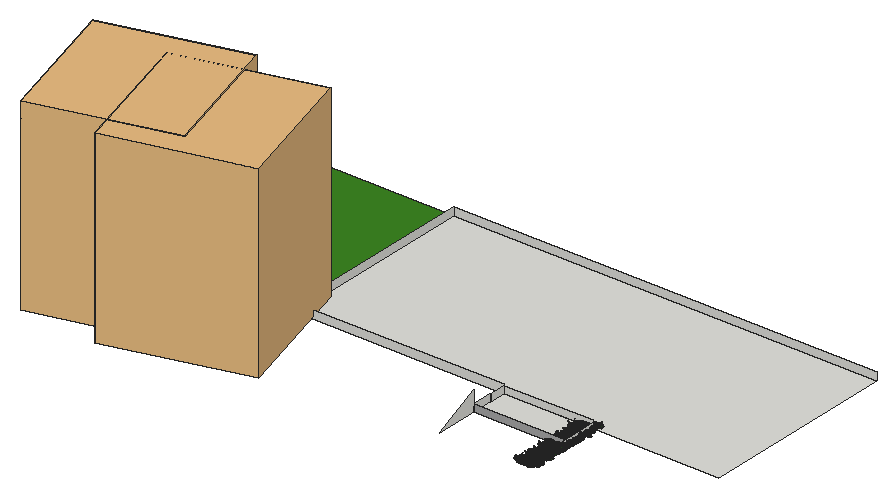
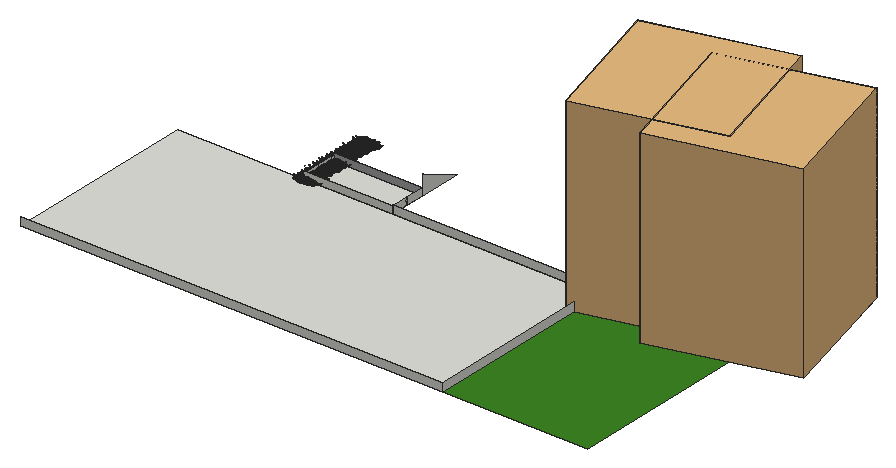
# SketchUp Ruby script. Lengths in inches.
U = 1.inch
M = Sketchup.active_model
def pt(a) = Geom::Point3d.new(a.map { |v| v * U })
def face(e, loops, mat)
  f = e.add_face(loops[0].map { |a| pt(a) })
  loops[1..].each { |l| e.add_face(l.map { |a| pt(a) }).erase! }
  f.material = f.back_material = mat if mat
  f
end
# faces: each face lists its corners as indices into pts; further lists are holes
def faces(e, pts, list, mat = nil) = list.each { |f| face(e, (f[0].is_a?(Array) ? f : [f]).map { |l| l.map { |i| pts[i] } }, mat) }
# xy, xz, yz: faces in a plane at the given z, y or x. An outline is a flat list of corners, or four numbers for a rectangle; further outlines are holes
def ring(l) = l.size == 4 ? [[l[0], l[1]], [l[2], l[1]], [l[2], l[3]], [l[0], l[3]]] : l.each_slice(2).to_a
def flat(e, list, mat, &to3) = list.each { |f| face(e, (f[0].is_a?(Array) ? f : [f]).map { |l| ring(l).map { |u, v| to3.(u, v) } }, mat) }
def xy(e, z, list, mat = nil) = flat(e, list, mat) { |x, y| [x, y, z] }
def xz(e, y, list, mat = nil) = flat(e, list, mat) { |x, z| [x, y, z] }
def yz(e, x, list, mat = nil) = flat(e, list, mat) { |y, z| [x, y, z] }
def lines(e, pts, list) = list.each { |a, b| e.add_line(pt(pts[a]), pt(pts[b])) }
# prism: a flat outline (further loops are holes) pulled along v
def prism(e, loops, v, mat = nil)
  f = face(e, loops, mat); d = Geom::Vector3d.new(v.map { |x| x * U })
  f.pushpull(f.normal.samedirection?(d) ? d.length : -d.length)
end
def box(e, o, s, mat = nil) = prism(e, [[o, [o[0] + s[0], o[1], o[2]], [o[0] + s[0], o[1] + s[1], o[2]], [o[0], o[1] + s[1], o[2]]]], [0, 0, s[2]], mat)
def at(x, y, z, deg = 0) = Geom::Transformation.translation(pt([x, y, z])) * Geom::Transformation.rotation(ORIGIN, Z_AXIS, deg.degrees)
def axes(o, x, y, z) = Geom::Transformation.new([*x, 0, *y, 0, *z, 0, *pt(o).to_a, 1])
def part(name) = M.definitions.add(name)
# library, detail: a bought-in or finely detailed component or shape, given as its bounding box
def library(name, o, s) = part(name).tap { |d| box(d.entities, o, s) }
def detail(e, o, s) = box(e.add_group.entities, o, s)
def put(e, d, t, mat = nil) = e.add_instance(d, t).tap { |i| i.material = mat if mat }
def group(e, t, mat = nil) = e.add_group.tap { |g| g.transformation = t; g.material = mat if mat }.entities
root = M.entities
M.materials.add("Material82").color = [68, 110, 58]
M.materials.add("Material83").color = [48, 90, 38]
M.materials.add("Material84").color = [68, 110, 48]
M.materials.add("Material85").color = [48, 90, 48]
M.materials.add("Material86").color = [58, 110, 58]
M.materials.add("Material87").color = [58, 90, 38]
M.materials.add("Material88").color = [68, 100, 58]
M.materials.add("Material89").color = [48, 100, 38]
M.materials.add("[Color M01]").color = [60, 133, 34]
M.materials.add("[Color M03]1").color = [170, 170, 170]
c1 = library("Palm tree",[-4.09,-4.52,0],[193.52,193.51,258.93])
c2 = part("Palm+Tree")
put(c2.entities,c1,at(25.51,-21.81,0,15))
c3 = library("Group\#612",[0,0,0],[32.91,53.52,103.45])
c4 = part("grass00")
p = [[-0.6875,0.15,0],[-0.56,0.08,5.52],[-0.04,0.03,2.76],[0.48,-0.02,0],[0.35,-0.02,5.52],[-0.1,-0.14,5.52],
  [-0.12,0.65,8.37],[-0.42,0.65,8.37]]
faces(c4.entities,p,[[0,1,2,3],[3,2,4],[1,5,2],[5,4,2],[1,6,5],[4,5,6],[7,6,1]])
c5 = part("Group16\#1")
put(c5.entities,c4,axes([1.44,-0.61,-0.01],[0.05352,0.12609,0],[-0.10704,0.04543,0.07239],[0.06664,-0.02828,0.11628]),"Material85")
put(c5.entities,c4,axes([0.76,-0.15,-0.01],[0.04676,0.24062,0],[-0.23162,0.04501,0.06642],[0.0652,-0.01267,0.23595]),"Material82")
put(c5.entities,c4,axes([0.79,0.01,-0.01],[-0.00606,0.34651,0],[-0.34381,-0.00602,0.0432],[0.04319,0.00076,0.34386]))
put(c5.entities,c4,axes([1,0.23,-0.01],[-0.07192,0.31144,0],[-0.28722,-0.06632,0.1236],[0.12043,0.02781,0.29478]),"Material84")
put(c5.entities,c4,axes([1.66,0.77,-0.01],[-0.13828,0.29651,0],[-0.21551,-0.1005,0.22471],[0.20365,0.09498,0.23779]),"Material89")
put(c5.entities,c4,axes([0.6875,0.52,-0.01],[-0.18126,0.24051,0],[-0.22746,-0.17142,0.09788],[0.07817,0.05891,0.28481]),"Material84")
put(c5.entities,c4,axes([0.68,0.78,-0.01],[-0.215,0.18688,0],[-0.12385,-0.14248,0.21334],[0.13995,0.16101,0.18878]),"Material82")
put(c5.entities,c4,axes([0.56,1,-0.01],[-0.13756,0.07624,0],[-0.06159,-0.11112,0.0927],[0.04494,0.08108,0.12705]),"Material84")
put(c5.entities,c4,axes([0.2,0.64,-0.01],[-0.23729,0.07254,0],[-0.05711,-0.18681,0.153],[0.04473,0.14632,0.19535]),"Material89")
put(c5.entities,c4,axes([0.0625,0.72,-0.01],[-0.28874,0.02525,0],[-0.02179,-0.24916,0.14647],[0.01276,0.14591,0.25012]),"Material82")
put(c5.entities,c4,axes([-0.08,0.62,-0.01],[-0.34089,-0.04187,0],[0.03255,-0.26504,0.216],[-0.02633,0.21439,0.26703]),"Material89")
put(c5.entities,c4,axes([-0.34,0.98,-0.01],[-0.14314,-0.0493,0],[0.04397,-0.12769,0.06843],[-0.02228,0.0647,0.13505]),"Material89")
put(c5.entities,c4,axes([-0.87,1.45,-0.01],[-0.23488,-0.14114,0],[0.13761,-0.22901,0.06087],[-0.03135,0.05217,0.26717]))
put(c5.entities,c4,axes([-0.72,0.77,-0.01],[-0.14208,-0.13251,0],[0.07209,-0.0773,0.16301],[-0.11118,0.11922,0.1057]),"Material89")
put(c5.entities,c4,axes([-0.62,0.43,-0.01],[-0.14845,-0.21203,0],[0.18654,-0.13061,0.12304],[-0.10079,0.07057,0.22772]),"Material82")
put(c5.entities,c4,axes([-0.68,0.29,-0.01],[-0.13639,-0.32136,0],[0.31723,-0.13464,0.05579],[-0.05136,0.0218,0.34462]),"Material83")
put(c5.entities,c4,axes([-0.64,0.125,-0.01],[-0.0458,-0.23569,0],[0.22124,-0.043,0.08276],[-0.08124,0.01579,0.22538]),"Material86")
put(c5.entities,c4,axes([-1.6,-0.03,-0.01],[0.00576,-0.32897,0],[0.27526,0.00482,0.18018],[-0.18015,-0.00315,0.2753]),"Material84")
put(c5.entities,c4,axes([-1.36,-0.31,-0.01],[0.05718,-0.24765,0],[0.18172,0.04196,0.17267],[-0.16825,-0.03885,0.1865]),"Material89")
put(c5.entities,c4,axes([-1.54,-0.72,-0.01],[0.06537,-0.14017,0],[0.13555,0.06321,0.03939],[-0.0357,-0.01665,0.14956]))
put(c5.entities,c4,axes([-1.19,-0.9,-0.01],[0.09597,-0.12735,0],[0.11214,0.08451,0.07557],[-0.06035,-0.04548,0.14042]),"Material88")
put(c5.entities,c4,axes([-0.47,-0.54,-0.01],[0.11588,-0.10072,0],[0.0618,0.0711,0.12124],[-0.07953,-0.0915,0.0942]))
put(c5.entities,c4,axes([-0.47,-0.84,-0.01],[0.11927,-0.0661,0],[0.06603,0.11913,0.00646],[-0.00313,-0.00565,0.13621]),"Material84")
put(c5.entities,c4,axes([-0.38,-1.24,-0.01],[0.28037,-0.08571,0],[0.0618,0.20215,0.20315],[-0.05939,-0.19428,0.21139]),"Material88")
put(c5.entities,c4,axes([-0.06,-0.66,-0.01],[0.22719,-0.01987,0],[0.01247,0.14255,0.17758],[-0.01547,-0.17691,0.1431]),"Material87")
put(c5.entities,c4,axes([0.11,-0.89,-0.01],[0.14882,0.01828,0],[-0.01058,0.08611,0.12229],[0.01491,-0.12138,0.08676]),"Material85")
put(c5.entities,c4,axes([0.25,-0.72,-0.01],[0.20481,0.07053,0],[-0.06206,0.18022,0.10291],[0.03351,-0.0973,0.1906]),"Material85")
put(c5.entities,c4,axes([0.85,-1.42,-0.01],[0.16481,0.09904,0],[-0.09472,0.15762,0.05616],[0.02893,-0.04814,0.18389]),"Material84")
put(c5.entities,c4,axes([1.01,-1.09,-0.01],[0.21858,0.20385,0],[-0.17495,0.1876,0.15339],[0.10462,-0.11218,0.25652]),"Material89")
put(c5.entities,c4,axes([1.01,-0.71,-0.01],[0.08733,0.12473,0],[-0.06445,0.04512,0.13037],[0.1068,-0.07477,0.07867]),"Material85")
c6 = part("Group15\#1")
put(c6.entities,c5,at(0,0,0))
c7 = part("3darcstudiotree_grass00\#1")
put(c7.entities,c6,at(0,0,0))
xy(root,-29.74,[[115.625,932.5,199.6875,932.62],[486.07,994.94,608.75,1046.93],[199.6875,1046.93,782.4375,1318.18]])
xy(root,-29.74,[[0,932.62,199.6875,1318.18]],"[Color M01]")
xz(root,994.94,[[486.07,-29.74,608.75,-19.8125]],"[Color M03]1")
xz(root,1046.93,[[199.6875,-29.74,208.57,-19.8125],[208.57,-29.74,486.07,-18.36],[486.07,-29.74,608.75,-19.8125]])
xz(root,1318.18,[[199.6875,-29.74,782.4375,-18.36]])
yz(root,199.6875,[[935.62,-29.74,994.94,-2.1875,994.94,-29.74],[994.94,-29.74,1046.93,-19.8125],[1046.93,-29.74,1318.18,-18.36]])
yz(root,486.07,[[935.62,-29.74,994.94,-29.74,994.94,-2.1875],[994.94,-29.74,1022.06,-19.8125],[1022.06,-29.74,1023.55,-19.8125],[1023.55,-29.74,1046.93,-19.8125]])
yz(root,608.75,[[994.94,-29.74,1000.12,-23.22],[1000.12,-29.74,1022.06,-23.22],[1022.06,-29.74,1046.93,-23.22]])
put(root,c2,at(-57.9,891.52,-29.74))
put(root,c3,axes([67.04,894.49,-29.74],[1.13014,0.75656,0],[-0.75656,1.13014,0],[0,0,1.36]))
put(root,c2,at(49.04,885.71,-29.74))
put(root,c7,axes([596.43,1010.04,-29.74],[-3.06097,-0.5879,0],[1.66705,-1.34995,-0.03924],[0.1162,-0.0941,1.93013]))
put(root,c7,axes([597.12,958.21,-29.74],[-1.33725,-1.41841,0],[4.13991,-0.60704,-0.02925],[0.14115,-0.0207,1.7044]))
put(root,c7,axes([597.16,946.84,-29.74],[-4.40805,-0.66258,0],[1.20213,-1.24385,-0.04688],[0.1049,-0.10854,1.58936]))
put(root,c7,axes([597.28,948.47,-29.74],[-4.593,-0.45536,0],[0.84159,-1.32024,-0.02201],[0.02791,-0.04378,1.34565]))
put(root,c7,axes([596.53,997.65,-29.74],[2.83648,-1.2359,0],[3.15131,1.12486,-0.01132],[0.04822,0.01721,1.83032]))
put(root,c7,axes([597.54,983.19,-29.74],[-1.4633,-1.68853,0],[3.81957,-0.51482,-0.03013],[0.1448,-0.01952,1.53631]))
put(root,c7,axes([597.5,1031.95,-29.74],[0.43217,-1.5656,0],[4.20709,0.18062,-0.01362],[0.0661,0.00284,1.54899]))
put(root,c7,axes([597.03,1035.85,-29.74],[-3.35215,0.96429,0],[-2.54913,-1.37823,-0.03459],[-0.11585,-0.06264,1.84283]))
put(root,c7,axes([596.27,940.12,-29.74],[3.65261,0,0],[0,1.44049,0],[0,0,1]))
put(root,c7,axes([598.06,1042.6,-29.74],[-1.52778,-1.4368,0],[3.26203,-0.53947,-0.00949],[0.054,-0.00893,1.63563]))
put(root,c7,axes([597,1044.86,-29.74],[-2.50316,1.24796,0],[-3.26881,-1.01974,-0.0328],[-0.10917,-0.03406,1.32564]))
put(root,c7,axes([598,1014.65,-29.74],[-4.03652,-0.16228,0],[0.44348,-1.71564,-0.03002],[0.01485,-0.05745,1.59842]))
put(root,c7,axes([596.5,982.15,-29.74],[3.25905,0.69762,0],[-2.04099,1.48295,-0.01651],[-0.04447,0.03231,1.81134]))
put(root,c7,axes([597.27,960.26,-29.74],[-1.85538,1.37845,0],[-3.32658,-0.69639,-0.02935],[-0.1215,-0.02544,1.32321]))
put(root,c7,axes([597.24,1051.48,-29.74],[-1.47744,1.354,0],[-3.50661,-0.5951,-0.01574],[-0.08407,-0.01427,1.66349]))
put(root,c7,axes([597.69,1019.44,-29.74],[2.89762,-1.1399,0],[2.43274,0.96179,-0.0036],[0.01556,0.00615,1.5794]))
put(root,c7,axes([597.16,992.45,-29.74],[-2.16254,1.46376,0],[-3.92939,-0.90288,-0.00219],[-0.00913,-0.0021,1.64693]))
put(root,c7,axes([596.89,1037.79,-29.74],[3.10066,0.47843,0],[-1.67535,1.68868,-0.03882],[-0.06401,0.06452,1.55956]))
put(root,c7,axes([597.33,951.63,-29.74],[3.24585,-0.20669,0],[0.57348,1.40067,-0.03713],[0.03058,0.07468,1.39317]))
put(root,c7,axes([597.91,1048.56,-29.74],[-2.59394,1.01102,0],[-3.072,-1.22583,-0.01852],[-0.05979,-0.02386,1.50457]))
put(root,c7,axes([597.61,1001.8,-29.74],[3.9501,-0.3019,0],[0.82816,1.68526,-0.01483],[0.01308,0.02661,1.51152]))
put(root,c7,axes([597.7,979.3,-29.74],[3.32132,-0.19382,0],[0.6507,1.73421,-0.00326],[0.00271,0.00722,1.88794]))
put(root,c7,axes([597.3,1023.55,-29.74],[3.35543,0.83331,0],[-2.02345,1.2672,-0.03908],[-0.13338,0.08353,1.82303]))
put(root,c7,axes([597.59,942.22,-29.74],[1.50682,1.6341,0],[-3.24176,0.46492,-0.03897],[-0.21712,0.03114,1.53286]))
put(root,c7,axes([598.04,1007.71,-29.74],[2.855,1.42821,0],[-2.79418,0.86872,-0.04305],[-0.19263,0.05989,1.51958]))
put(root,c7,axes([599.67,986.04,-29.74],[-4.71763,0.13616,0],[-0.3116,-1.67918,-0.0067],[-0.002,-0.01078,1.30916]))
put(root,c7,axes([599.57,992.48,-29.74],[0.36596,-1.66077,0],[4.11633,0.14107,-0.03115],[0.15736,0.00539,1.5702]))
put(root,c7,axes([600.12,988.04,-29.74],[1.0844,-1.46677,0],[3.4842,0.40063,-0.01207],[0.07085,0.00815,1.66287]))
put(root,c7,axes([600.5,1045.3125,-29.74],[-3.58141,-0.41852,0],[1.07572,-1.43168,-0.05017],[0.07746,-0.10309,1.54202]))
put(root,c7,axes([600.92,1036.04,-29.74],[-2.10821,-1.47996,0],[3.50963,-0.77757,-0.0488],[0.18715,-0.04146,1.32723]))
put(root,c7,axes([600.35,942.81,-29.74],[2.27608,-1.0007,0],[3.35316,1.18618,-0.03873],[0.1622,0.05738,1.89965]))
put(root,c7,axes([600.82,972.67,-29.74],[-3.59463,0.44793,0],[-1.16817,-1.45801,-0.02199],[-0.03431,-0.04283,1.50537]))
put(root,c7,axes([600.8,968.48,-29.74],[2.73821,-1.25836,0],[3.57659,1.21044,-0.00643],[0.02336,0.00791,1.6911]))
put(root,c7,axes([599.74,1030.12,-29.74],[4.14496,0.31804,0],[-0.83759,1.6978,-0.03864],[-0.04159,0.0843,1.85268]))
put(root,c7,axes([599.96,998.79,-29.74],[4.22455,0.00563,0],[-0.01154,1.34671,-0.00416],[-0.00007,0.00858,1.3392]))
put(root,c7,axes([599.91,1001.3125,-29.74],[3.14768,1.20624,0],[-3.13864,1.27383,-0.06236],[-0.23969,0.09728,1.86199]))
put(root,c7,axes([601.71,1051.8125,-29.74],[-2.67553,-0.98375,0],[2.79136,-1.18074,-0.04642],[0.15585,-0.06593,1.51042]))
put(root,c7,axes([601.24,1026.87,-29.74],[1.22629,-1.22817,0],[3.78204,0.58732,-0.0431],[0.18193,0.02825,1.38217]))
put(root,c7,axes([600.11,989.92,-29.74],[-0.387,1.5813,0],[-4.71042,-0.17929,-0.01578],[-0.06068,-0.00231,1.37044]))
put(root,c7,axes([601.28,1013.93,-29.74],[2.09831,-1.02697,0],[3.53268,1.1226,-0.04335],[0.15343,0.04876,1.54559]))
put(root,c7,axes([601.91,1043.03,-29.74],[-1.12016,-1.49158,0],[3.32126,-0.38792,-0.01669],[0.11216,-0.0131,1.82011]))
put(root,c7,axes([601.16,1010.39,-29.74],[-2.72452,1.24598,0],[-3.55259,-1.2082,-0.04683],[-0.18808,-0.06396,1.86493]))
put(root,c7,axes([600.16,958.07,-29.74],[0.67723,1.39261,0],[-4.43088,0.33513,-0.00068],[-0.00322,0.00024,1.62852]))
put(root,c7,axes([601.62,976.62,-29.74],[1.58844,-1.66939,0],[3.21642,0.47599,-0.02337],[0.14197,0.02101,1.67088]))
put(root,c7,axes([601.98,946.1,-29.74],[-3.67612,0.09043,0],[-0.28445,-1.79854,-0.0193],[-0.00469,-0.02963,1.33558]))
put(root,c7,axes([600.94,944.87,-29.74],[0.19969,1.44757,0],[-3.37153,0.07234,-0.03311],[-0.18886,0.00405,1.44579]))
put(root,c7,axes([602.25,1040.18,-29.74],[-3.74626,-0.28421,0],[0.67953,-1.39309,-0.01319],[0.01627,-0.03336,1.76124]))
put(root,c7,axes([600.64,1016.4,-29.74],[3.77194,0.53127,0],[-1.56854,1.73204,-0.02984],[-0.04464,0.0493,1.55474]))
put(root,c7,axes([602.32,994.86,-29.74],[0.06282,-1.34984,0],[3.50326,0.02536,-0.01436],[0.0861,0.00062,1.57494]))
put(root,c7,axes([602.27,1012.27,-29.74],[0.71144,-1.32945,0],[4.31841,0.35942,-0.04294],[0.17046,0.01419,1.34209]))
put(root,c7,axes([601.51,948.1,-29.74],[-2.51102,1.11498,0],[-3.04783,-1.06754,-0.01682],[-0.06435,-0.02254,1.56312]))
put(root,c7,axes([602.81,1046.51,-29.74],[-4.08051,-0.34509,0],[0.80518,-1.48079,-0.03168],[0.03378,-0.06213,1.46389]))
put(root,c7,axes([602.43,982,-29.74],[-3.50605,0.34582,0],[-0.87343,-1.37724,-0.00789],[-0.01222,-0.01927,1.7222]))
put(root,c7,axes([602.56,1019.35,-29.74],[1.7149,-1.22637,0],[3.67075,0.79833,-0.00061],[0.00329,0.00072,1.94394]))
put(root,c7,axes([601.32,951.68,-29.74],[4.50029,0.14913,0],[-0.32235,1.51291,-0.00911],[-0.00515,0.02417,1.94776]))
put(root,c7,axes([602.89,1021.36,-29.74],[1.13517,-1.33714,0],[4.08386,0.53922,-0.04023],[0.16123,0.02129,1.36415]))
put(root,c7,axes([601.97,1025.36,-29.74],[-1.96155,1.42232,0],[-3.86474,-0.82896,-0.01158],[-0.04562,-0.00979,1.47884]))
put(root,c7,axes([602.54,975.37,-29.74],[-3.11045,1.07931,0],[-2.57078,-1.15227,-0.02195],[-0.09054,-0.04058,1.82186]))
put(root,c7,axes([603.37,1031.55,-29.74],[-0.47401,-1.83018,0],[3.81106,-0.15352,-0.01024],[0.06486,-0.00261,1.82793]))
put(root,c7,axes([603.01,980.125,-29.74],[2.67895,-1.42027,0],[3.76202,1.10364,-0.01386],[0.04132,0.01212,1.30579]))
put(root,c7,axes([603.58,964.375,-29.74],[-4.02887,-0.32689,0],[0.86941,-1.66657,-0.02294],[0.02463,-0.04722,1.72347]))
put(root,c7,axes([602.59,959.83,-29.74],[3.37179,-0.80655,0],[2.39395,1.55652,-0.03972],[0.09789,0.06365,1.6444]))
put(root,c7,axes([601.82,983.55,-29.74],[3.19117,1.02249,0],[-2.28557,1.10943,-0.0068],[-0.02189,0.01063,1.38619]))
put(root,c7,axes([601.9,966.21,-29.74],[0.53207,1.56479,0],[-4.35061,0.23008,-0.0098],[-0.05087,0.00269,1.72283]))
put(root,c7,axes([602.03,971.08,-29.74],[3.6725,0.99677,0],[-2.44181,1.39924,-0.05897],[-0.19798,0.11345,1.91169]))
put(root,c7,axes([602.82,997.62,-29.74],[-1.969,1.11609,0],[-3.42444,-0.93961,-0.02835],[-0.10891,-0.02988,1.46355]))
put(root,c7,axes([602.18,1034.3125,-29.74],[-0.22309,1.29668,0],[-4.38525,-0.11734,-0.00038],[-0.00168,-0.00004,1.44006]))
put(root,c7,axes([603.32,954.59,-29.74],[-3.28336,1.15138,0],[-2.69769,-1.19648,-0.01814],[-0.06877,-0.0305,1.73642]))
put(root,c7,axes([602.5,1037.56,-29.74],[2.78968,1.01154,0],[-2.64,1.13236,-0.04265],[-0.18761,0.08047,1.90027]))
put(root,c7,axes([602.79,1023,-29.74],[-2.22727,1.60419,0],[-4.12877,-0.89155,-0.00813],[-0.02667,-0.00576,1.31962]))
put(root,c7,axes([603.14,1007.45,-29.74],[-2.60888,1.40075,0],[-3.4553,-1.0009,-0.02364],[-0.11495,-0.0333,1.93862]))
put(root,c7,axes([603.52,1006.35,-29.74],[3.43972,-1.19732,0],[3.07284,1.37298,-0.00351],[0.01073,0.00479,1.60808]))
put(root,c7,axes([603.45,962.37,-29.74],[-2.75837,1.17724,0],[-3.35186,-1.22148,-0.01856],[-0.07358,-0.02681,1.84646]))
put(root,c7,axes([603.54,1004.03,-29.74],[2.57433,-1.10368,0],[3.03991,1.10279,-0.05921],[0.27011,0.09799,1.91907]))
put(root,c7,axes([603.07,940.17,-29.74],[4.03336,-0.1179,0],[0.28483,1.51556,-0.02045],[0.00943,0.05018,1.8024]))
put(root,c7,axes([603.55,1049.3125,-29.74],[-2.1063,1.53486,0],[-3.86767,-0.82549,-0.04902],[-0.23106,-0.04932,1.76654]))
put(root,c7,axes([605.46,1023.5,-29.74],[-1.00872,-1.50256,0],[3.76018,-0.39261,-0.00114],[0.00668,-0.0007,1.77079]))
put(root,c7,axes([603.54,953.76,-29.74],[1.54692,1.35045,0],[-3.5946,0.6404,-0.01637],[-0.06936,0.01236,1.37485]))
put(root,c7,axes([605.11,987.9,-29.74],[-1.02138,-1.60708,0],[3.36091,-0.33222,-0.0349],[0.24018,-0.02374,1.84282]))
put(root,c7,axes([605.75,1010.12,-29.74],[-4.39065,-0.68044,0],[1.48247,-1.48779,-0.03326],[0.06181,-0.06203,1.54402]))
put(root,c7,axes([605.74,1024.88,-29.74],[-4.44259,0.07323,0],[-0.15396,-1.45277,-0.02048],[-0.00618,-0.05831,1.99696]))
put(root,c7,axes([605.25,1020.67,-29.74],[-2.76199,0.84111,0],[-2.40625,-1.22891,-0.02049],[-0.06035,-0.03082,1.42185]))
put(root,c7,axes([606.14,948.87,-29.74],[-4.39876,-0.08421,0],[0.22064,-1.79246,-0.01036],[0.00206,-0.01674,1.39846]))
put(root,c7,axes([605.75,1036.34,-29.74],[2.13524,-1.29449,0],[3.0122,0.77275,-0.01966],[0.10051,0.02579,1.64285]))
put(root,c7,axes([606.47,975.56,-29.74],[-2.27298,-1.15312,0],[2.90139,-0.88948,-0.04864],[0.26323,-0.0807,1.88819]))
put(root,c7,axes([606.45,957.29,-29.74],[-0.27323,-1.39515,0],[4.04907,-0.12333,-0.04603],[0.24308,-0.0074,1.61216]))
put(root,c7,axes([605.94,995.35,-29.74],[-3.30373,1.03648,0],[-2.84639,-1.41107,-0.00639],[-0.01873,-0.00928,1.6128]))
put(root,c7,axes([606.94,977.95,-29.74],[-4.23108,-0.20575,0],[0.45076,-1.44167,-0.03319],[0.02288,-0.07317,1.55524]))
put(root,c7,axes([606.38,1044.59,-29.74],[-2.75278,0.82906,0],[-2.65464,-1.37089,-0.0597],[-0.21369,-0.11035,1.93343]))
put(root,c7,axes([605.93,1049.82,-29.74],[-1.7142,1.30326,0],[-3.68982,-0.75483,-0.04385],[-0.17675,-0.03616,1.41492]))
put(root,c7,axes([606.43,1037.99,-29.74],[-2.52665,1.52426,0],[-3.1276,-0.80632,-0.05029],[-0.29899,-0.07708,1.98932]))
put(root,c7,axes([606.75,1033.74,-29.74],[1.00905,-1.48256,0],[4.12419,0.43657,-0.05256],[0.2523,0.02671,1.59089]))
put(root,c7,axes([607.25,991.87,-29.74],[-1.34868,-1.52366,0],[4.27,-0.58784,-0.05387],[0.21958,-0.03023,1.46363]))
put(root,c7,axes([607.19,1042.67,-29.74],[-0.81771,-1.39799,0],[3.86882,-0.35195,-0.03351],[0.1754,-0.01596,1.59864]))
put(root,c7,axes([605.85,1003.57,-29.74],[4.22079,-0.16227,0],[0.44484,1.79962,-0.00515],[0.00263,0.01065,1.80879]))
put(root,c7,axes([605.91,966.15,-29.74],[3.56541,-0.13016,0],[0.37676,1.60514,-0.05657],[0.02546,0.10845,1.49576]))
put(root,c7,axes([606.73,968.125,-29.74],[-3.05652,0.90078,0],[-1.97442,-1.04198,-0.01872],[-0.07362,-0.03885,1.62421]))
put(root,c7,axes([606.92,945.04,-29.74],[-3.18956,0.31713,0],[-1.10467,-1.728,-0.01943],[-0.01876,-0.02934,1.33771]))
put(root,c7,axes([607.47,981.1,-29.74],[-3.13974,-0.75675,0],[2.02292,-1.30536,-0.04274],[0.1274,-0.08221,1.66217]))
put(root,c7,axes([607.6,985.7,-29.74],[-4.11825,0.06325,0],[-0.12995,-1.31605,-0.00954],[-0.0021,-0.02124,1.41434]))
put(root,c7,axes([606.72,983.48,-29.74],[-0.62058,1.51993,0],[-3.60511,-0.22893,-0.03829],[-0.23497,-0.01492,1.70109]))
put(root,c7,axes([607.96,1000.55,-29.74],[-4.16244,-0.15093,0],[0.36502,-1.56574,-0.01686],[0.00714,-0.03063,1.38194]))
put(root,c7,axes([608.125,972.77,-29.74],[-0.89443,-1.66932,0],[4.23179,-0.35265,-0.02196],[0.11928,-0.00994,1.79942]))
put(root,c7,axes([606.34,963.48,-29.74],[2.80483,0.78712,0],[-2.29694,1.27299,-0.00585],[-0.01927,0.01068,1.68777]))
put(root,c7,axes([607.77,951.6875,-29.74],[1.02165,-1.42104,0],[3.23224,0.36142,-0.01712],[0.09227,0.01032,1.41054]))
put(root,c7,axes([606.64,1017.22,-29.74],[-0.6643,1.32662,0],[-4.47997,-0.3489,-0.01512],[-0.08059,-0.00628,1.85999]))
put(root,c7,axes([608.21,1008.36,-29.74],[0.943,-1.41783,0],[3.80413,0.39351,-0.01105],[0.05525,0.00572,1.52421]))
put(root,c7,axes([608.53,962.71,-29.74],[-4.34806,-0.2749,0],[0.62437,-1.53594,-0.05495],[0.04724,-0.1162,1.60563]))
put(root,c7,axes([606.77,999.22,-29.74],[0.93193,1.68006,0],[-3.63506,0.3136,-0.00261],[-0.01526,0.00132,1.6704]))
put(root,c7,axes([606.76,1032.11,-29.74],[2.55431,1.01117,0],[-3.10398,1.2195,-0.03194],[-0.09397,0.03692,1.36388]))
put(root,c7,axes([608.17,996.35,-29.74],[1.68936,-1.29831,0],[3.68445,0.74564,-0.0206],[0.10358,0.02096,1.75423]))
put(root,c7,axes([608.39,970.65,-29.74],[0.80832,-1.39105,0],[3.86121,0.34896,-0.01662],[0.09893,0.00894,1.81323]))
put(root,c7,axes([607.2,960.375,-29.74],[1.77276,1.31188,0],[-3.2596,0.68507,-0.05193],[-0.30681,0.06448,1.85357]))
put(root,c7,axes([608.84,1014.65,-29.74],[-3.93808,-0.75827,0],[2.05575,-1.66052,-0.06565],[0.13947,-0.11266,1.70067]))
put(root,c7,axes([609.05,1051.76,-29.74],[-1.23898,-1.77649,0],[4.18164,-0.45359,-0.02011],[0.11729,-0.01272,1.9663]))
put(root,c7,axes([607.24,1018.35,-29.74],[-0.07538,1.68656,0],[-4.43832,-0.03085,-0.00958],[-0.0427,-0.0003,1.48335]))
put(root,c7,axes([608.75,978.6,-29.74],[0.5287,-1.47174,0],[3.5141,0.19634,-0.02485],[0.18259,0.0102,1.97391]))
put(root,c7,axes([607.61,1039.76,-29.74],[4.04964,0.85012,0],[-2.04869,1.51784,-0.02998],[-0.08539,0.06326,1.98098]))
put(root,c7,axes([608.07,1006.2,-29.74],[0.31598,1.50106,0],[-3.48689,0.11416,-0.00998],[-0.05116,0.00168,1.34846]))
put(root,c7,axes([608.64,941.81,-29.74],[3.14916,-0.41283,0],[1.21857,1.44573,-0.00205],[0.00401,0.00476,1.79239]))
put(root,c7,axes([608.89,1030.27,-29.74],[3.02082,-1.15648,0],[2.42176,0.98385,-0.02978],[0.11407,0.04634,1.43312]))
put(root,c7,axes([608.72,946.47,-29.74],[-1.68906,1.71794,0],[-3.99186,-0.61041,-0.03012],[-0.15949,-0.02439,1.82227]))
